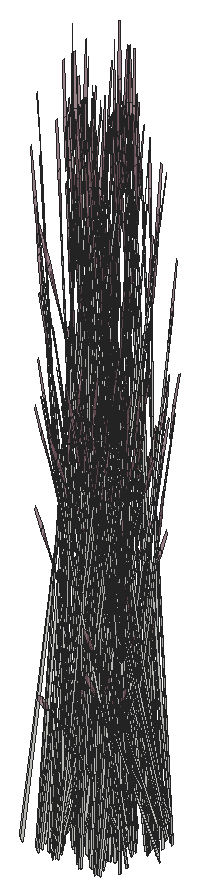
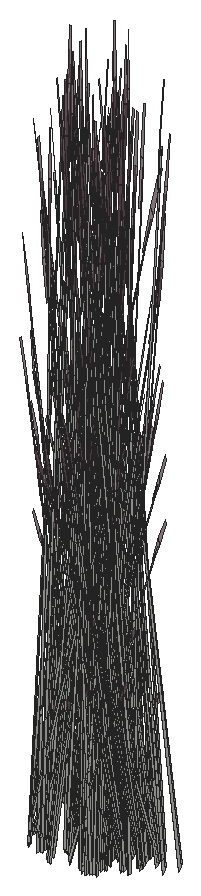
# SketchUp Ruby script. Lengths in inches.
U = 1.inch
M = Sketchup.active_model
def pt(a) = Geom::Point3d.new(a.map { |v| v * U })
def face(e, loops, mat)
  f = e.add_face(loops[0].map { |a| pt(a) })
  loops[1..].each { |l| e.add_face(l.map { |a| pt(a) }).erase! }
  f.material = f.back_material = mat if mat
  f
end
# faces: each face lists its corners as indices into pts; further lists are holes
def faces(e, pts, list, mat = nil) = list.each { |f| face(e, (f[0].is_a?(Array) ? f : [f]).map { |l| l.map { |i| pts[i] } }, mat) }
# xy, xz, yz: faces in a plane at the given z, y or x. An outline is a flat list of corners, or four numbers for a rectangle; further outlines are holes
def ring(l) = l.size == 4 ? [[l[0], l[1]], [l[2], l[1]], [l[2], l[3]], [l[0], l[3]]] : l.each_slice(2).to_a
def flat(e, list, mat, &to3) = list.each { |f| face(e, (f[0].is_a?(Array) ? f : [f]).map { |l| ring(l).map { |u, v| to3.(u, v) } }, mat) }
def xy(e, z, list, mat = nil) = flat(e, list, mat) { |x, y| [x, y, z] }
def xz(e, y, list, mat = nil) = flat(e, list, mat) { |x, z| [x, y, z] }
def yz(e, x, list, mat = nil) = flat(e, list, mat) { |y, z| [x, y, z] }
def lines(e, pts, list) = list.each { |a, b| e.add_line(pt(pts[a]), pt(pts[b])) }
# prism: a flat outline (further loops are holes) pulled along v
def prism(e, loops, v, mat = nil)
  f = face(e, loops, mat); d = Geom::Vector3d.new(v.map { |x| x * U })
  f.pushpull(f.normal.samedirection?(d) ? d.length : -d.length)
end
def box(e, o, s, mat = nil) = prism(e, [[o, [o[0] + s[0], o[1], o[2]], [o[0] + s[0], o[1] + s[1], o[2]], [o[0], o[1] + s[1], o[2]]]], [0, 0, s[2]], mat)
def at(x, y, z, deg = 0) = Geom::Transformation.translation(pt([x, y, z])) * Geom::Transformation.rotation(ORIGIN, Z_AXIS, deg.degrees)
def axes(o, x, y, z) = Geom::Transformation.new([*x, 0, *y, 0, *z, 0, *pt(o).to_a, 1])
def part(name) = M.definitions.add(name)
# library, detail: a bought-in or finely detailed component or shape, given as its bounding box
def library(name, o, s) = part(name).tap { |d| box(d.entities, o, s) }
def detail(e, o, s) = box(e.add_group.entities, o, s)
def put(e, d, t, mat = nil) = e.add_instance(d, t).tap { |i| i.material = mat if mat }
def group(e, t, mat = nil) = e.add_group.tap { |g| g.transformation = t; g.material = mat if mat }.entities
root = M.entities
M.materials.add("LightPink_Translucent").color = [144, 107, 117]
M.materials["LightPink_Translucent"].alpha = 0.75
c1 = part("blade")
p = [[2.15,0.21,22],[0,0.17,0],[0.09,0.45,0],[2.18,0.31,22],[2.29,0.31,22],[0.38,0.45,0],
  [2.48,0.24,33],[2.49,0.24,33],[2.48,0.22,33]]
faces(c1.entities,p,[[0,1,2,3],[4,5,2,3],[6,3,4,7],[8,0,3,6]])
c2 = part("seeds")
p = [[0.3,-0.1,1.38],[-0.01,-0.03,1.59],[-0.01,-0.03,0.03],[0.14,-0.07,-0.07],[0.29,-0.03,3],[0.15,0.01,3.11]]
faces(c2.entities,p,[[0,1,2,3],[1,0,4,5]],"LightPink_Translucent")
c3 = part("blade with seeds")
put(c3.entities,c1,at(0,0,0))
put(c3.entities,c2,axes([2.4,0.25,30.99],[1.5799,-0.05474,1.17369],[-0.12525,1.92788,0.29478],[-0.07173,-0.02425,1.56792]))
put(root,c3,axes([356.83,652.4,625.22],[-0.1064,0.35863,0.35414],[-0.31043,-0.1046,-0.4572],[-0.02846,-0.14439,0.87481]))
put(root,c3,axes([350.33,651.97,625.26],[-0.17758,-0.42229,-0.1216],[0.31518,-0.20752,-0.67495],[0.13282,-0.05572,1.02557]))
put(root,c3,axes([350.32,651.6,624.91],[0.09562,-0.42421,-0.51099],[0.32782,0.1454,-0.3958],[0.13199,-0.0389,0.97773]))
put(root,c3,axes([352.76,650.92,621.17],[0.32928,0.11539,-0.30978],[-0.08291,0.40636,0.30978],[0.06638,-0.04686,1.38974]))
put(root,c3,axes([349.8,649.875,622.6],[0.22066,-0.46731,0],[0.36918,0.26061,-0.51607],[0.08408,0.05936,1.63711]))
put(root,c3,axes([355.87,652.46,624.85],[-0.34827,0.11086,-0.51099],[-0.06092,-0.41983,-0.3958],[-0.09354,-0.12031,0.97773]))
put(root,c3,axes([356.11,652.09,625.6],[-0.23555,0.44708,-0.13619],[-0.34112,-0.25757,-0.75594],[-0.11858,-0.12631,1.14864]))
put(root,c3,axes([350.67,651.72,622.21],[-0.22732,0.05597,1.41583],[-0.03618,-0.44548,0.08104],[0.15921,-0.06743,0.80566]))
put(root,c3,axes([351.08,651.33,622.49],[-0.21881,-0.29821,-0.06488],[0.23965,-0.27324,-0.29416],[0.0679,-0.01924,0.97024]))
put(root,c3,axes([351.52,652.2,624.73],[-0.17758,-0.42229,-0.1216],[0.31518,-0.20752,-0.67495],[0.13282,-0.05572,1.02557]))
put(root,c3,axes([351.51,651.84,624.37],[0.09562,-0.42421,-0.51099],[0.32782,0.1454,-0.3958],[0.13199,-0.0389,0.97773]))
put(root,c3,axes([350.99,650.11,622.07],[0.22066,-0.46731,0],[0.36918,0.26061,-0.51607],[0.08408,0.05936,1.63711]))
put(root,c3,axes([354.65,651.92,623.87],[0.2423,0.19613,0.0643],[-0.14107,0.2793,0.50621],[0.07768,-0.0903,0.77189]))
put(root,c3,axes([354.58,651.84,623.87],[0.08753,0.42921,0.48003],[-0.34336,0.07449,0.3958],[0.1012,-0.10094,0.9933]))
put(root,c3,axes([356.42,651.83,622.3],[-0.2439,0.26754,-0.03893],[-0.22348,-0.29302,-0.17649],[-0.01573,-0.08303,0.58215]))
put(root,c3,axes([350.25,651.76,625.21],[0.31014,-0.20596,-0.71045],[0.17284,0.42397,0.08574],[0.14985,-0.04816,1.00501]))
put(root,c3,axes([351.86,651.96,621.67],[-0.22732,0.05597,1.41583],[-0.03618,-0.44548,0.08104],[0.15921,-0.06743,0.80566]))
put(root,c3,axes([352.27,651.57,621.95],[-0.21881,-0.29821,-0.06488],[0.23965,-0.27324,-0.29416],[0.0679,-0.01924,0.97024]))
put(root,c3,axes([358.3,652.55,625.55],[-0.00658,0.0559,1.77383],[-0.32474,0.20287,-0.16761],[-0.09556,-0.1037,0.31391]))
put(root,c3,axes([351.83,652.33,621.47],[-0.32829,0.39208,0.30756],[-0.32849,-0.38796,-0.36492],[-0.01146,-0.11134,1.64885]))
put(root,c3,axes([355.21,651.96,624.88],[-0.07594,-0.00329,1.74944],[-0.24177,0.32918,-0.27667],[-0.129,-0.06726,0.14031]))
put(root,c3,axes([350.8,650.36,622.17],[-0.33032,-0.23318,0.49651],[0.19744,-0.41812,0],[0.07523,0.05311,1.57504]))
put(root,c3,axes([351.45,652,624.67],[0.31014,-0.20596,-0.71045],[0.17284,0.42397,0.08574],[0.14985,-0.04816,1.00501]))
put(root,c3,axes([350.21,651.84,625.28],[-0.29332,-0.1301,0.35414],[0.08555,-0.37955,-0.4572],[0.11809,-0.0348,0.87481]))
put(root,c3,axes([352.87,652.52,621.57],[0.39767,0.22603,0.24065],[-0.19139,0.46966,0.50002],[0,-0.10827,1.60543]))
put(root,c3,axes([352.72,653.15,621.58],[0.09355,-0.55261,-0.23429],[0.44354,0.09633,0.51271],[-0.0775,-0.07631,1.5644]))
put(root,c3,axes([356.73,655,623.49],[0.305,0.18805,1.51261],[-0.29879,0.40513,0.59816],[-0.13384,-0.24012,1.26806]))
put(root,c3,axes([348.2,650.71,621.82],[-0.3474,0.18671,1.28929],[-0.11057,-0.53572,0.50096],[0.21332,0.00891,1.46642]))
put(root,c3,axes([356.09,652.46,625.22],[0.05451,0.37564,0.35414],[-0.31161,0.09919,-0.4572],[-0.0837,-0.10765,0.87481]))
put(root,c3,axes([355.13,653.7,622.1875],[0,-0.46636,-0.49651],[0.39487,0,0],[0,-0.10622,1.57504]))
put(root,c3,axes([355.15,652.7,625.26],[0.29147,-0.34417,0.53763],[0.25138,0.3655,0.4433],[-0.13675,-0.06349,1.11249]))
put(root,c3,axes([358.29,653.98,625.83],[-0.30095,-0.22541,-0.71045],[0.21388,-0.395,0.08574],[-0.10904,-0.13459,1.00501]))
put(root,c3,axes([350.91,651.43,621.72],[-0.01845,-0.0708,1.76342],[0.12793,-0.41416,-0.26939],[0.12905,-0.00596,0.30037]))
put(root,c3,axes([358.1875,653.68,625.37],[-0.05451,-0.37564,-0.35414],[0.31161,-0.09919,0.4572],[-0.0837,-0.10765,0.87481]))
put(root,c3,axes([351.4,652.08,624.74],[-0.29332,-0.1301,0.35414],[0.08555,-0.37955,-0.4572],[0.11809,-0.0348,0.87481]))
put(root,c3,axes([349.39,650.94,621.28],[-0.3474,0.18671,1.28929],[-0.11057,-0.53572,0.50096],[0.21332,0.00891,1.46642]))
put(root,c3,axes([352.74,652.2,621.86],[-0.38326,0.02879,0.44739],[-0.03466,-0.47788,-0.21531],[0.06861,-0.04843,1.43643]))
put(root,c3,axes([350.33,651.08,622.31],[0.06809,-0.4162,0.1448],[0.33266,0.07225,-0.41347],[0.06054,0.04274,1.26744]))
put(root,c3,axes([351.75,652.55,621.62],[0,0.46636,0.49651],[-0.39487,0,0],[0,-0.10622,1.57504]))
put(root,c3,axes([354.54,653.02,624.17],[-0.17758,-0.42229,-0.1216],[0.31518,-0.20752,-0.67495],[0.13282,-0.05572,1.02557]))
put(root,c3,axes([352.11,651.67,621.18],[-0.01845,-0.0708,1.76342],[0.12793,-0.41416,-0.26939],[0.12905,-0.00596,0.30037]))
put(root,c3,axes([354.01,650.93,621.51],[0.22066,-0.46731,0],[0.36918,0.26061,-0.51607],[0.08408,0.05936,1.63711]))
put(root,c3,axes([352.6875,652.93,621.35],[-0.21202,-0.39143,-0.44739],[0.32115,-0.27564,0.21531],[-0.06861,-0.04843,1.43643]))
put(root,c3,axes([352.73,652.375,621.5],[0.15345,0.52148,0.45755],[-0.43845,0.18134,0.17955],[0.00536,-0.09582,1.58856]))
put(root,c3,axes([349.1,650.98,622.89],[0.35635,-0.30962,-0.29095],[0.23697,0.43749,-0.50002],[0.08792,0.04443,1.59708]))
put(root,c3,axes([350.52,651.8,624.75],[0.29332,0.1301,-0.35414],[-0.08555,0.37955,0.4572],[0.11809,-0.0348,0.87481]))
put(root,c3,axes([350.19,651.19,622.41],[-0.21202,-0.39143,0.44739],[0.32115,-0.27564,-0.21531],[0.06861,0.04843,1.43643]))
put(root,c3,axes([355.28,652.7,624.9],[0.01777,-0.35463,0.0643],[0.26836,0.00972,0.50621],[-0.1028,-0.03711,0.77189]))
put(root,c3,axes([357.7,653.61,622.34],[-0.03419,0.06144,1.76342],[-0.3455,0.13246,-0.26939],[-0.08346,-0.12049,0.30037]))
put(root,c3,axes([350,650.16,622.24],[0.33032,0.23318,-0.49651],[-0.19744,0.41812,0],[0.07523,0.05311,1.57504]))
put(root,c3,axes([355.29,652.38,621.4],[-0.21881,-0.29821,-0.06488],[0.23965,-0.27324,-0.29416],[0.0679,-0.01924,0.97024]))
put(root,c3,axes([356.21,653.89,622.38],[0.17124,-0.42022,-0.44739],[0.35581,0.20224,0.21531],[0,-0.09687,1.43643]))
put(root,c3,axes([355.18,652.8125,624.7],[-0.20082,-0.29199,-0.35414],[0.2293,-0.2764,0.4572],[-0.1165,-0.04206,0.87481]))
put(root,c3,axes([352.65,652.78,621.86],[-0.17124,0.42022,0.44739],[-0.35581,-0.20224,-0.21531],[0,-0.09687,1.43643]))
put(root,c3,axes([353.28,652.42,621.34],[0,-0.53961,0],[0.44133,0,0],[0,0,1.79456]))
put(root,c3,axes([355.3,653.71,622.2],[0.24637,-0.29097,-0.30978],[0.24637,0.29097,0.30978],[0,-0.09372,1.38974]))
put(root,c3,axes([357.52,654.22,624.72],[0.1311,0.08035,1.71376],[-0.27131,0.33708,0.13857],[-0.16909,-0.15206,0.73262]))
put(root,c3,axes([350.29,651.22,622.36],[0.35635,-0.30962,-0.29095],[0.23697,0.43749,-0.50002],[0.08792,0.04443,1.59708]))
put(root,c3,axes([351.71,652.03,624.22],[0.29332,0.1301,-0.35414],[-0.08555,0.37955,0.4572],[0.11809,-0.0348,0.87481]))
put(root,c3,axes([353.82,651.17,621.62],[-0.33032,-0.23318,0.49651],[0.19744,-0.41812,0],[0.07523,0.05311,1.57504]))
put(root,c3,axes([355.2,652.32,622.3],[-0.10181,0.3808,-0.03893],[-0.31336,-0.11714,-0.17649],[-0.04758,-0.06228,0.58215]))
put(root,c3,axes([356.17,654.24,622.83],[-0.39748,-0.22252,-0.29095],[0.19139,-0.46966,-0.50002],[-0.01249,-0.11531,1.59708]))
put(root,c3,axes([349.72,651.33,624.1],[-0.14639,0.01056,1.71376],[0.09712,-0.45778,0.13857],[0.20862,0.02831,0.73262]))
put(root,c3,axes([351.19,650.4,621.71],[0.33032,0.23318,-0.49651],[-0.19744,0.41812,0],[0.07523,0.05311,1.57504]))
put(root,c3,axes([349.91,650.33,622.25],[0.08291,0.40636,-0.30978],[-0.32928,0.11539,0.30978],[0.06638,0.04686,1.38974]))
put(root,c3,axes([355.03,654.05,622.54],[-0.44133,0,0],[0,-0.52122,-0.51607],[0,-0.11871,1.63711]))
put(root,c3,axes([350.57,651.73,621.9],[0.39487,0,0],[0,0.48281,0],[0,0,1.78407]))
put(root,c3,axes([353.07,652.08,621.5],[-0.29264,0.42323,0.45755],[-0.34767,-0.3736,0.17955],[0.07055,-0.04224,1.58856]))
put(root,c3,axes([355.11,653.125,622.76],[0.06891,0.12984,1.43002],[-0.15879,0.35293,-0.30754],[-0.16304,-0.08436,0.61141]))
put(root,c3,axes([358.15,653.99,625.53],[-0.34827,0.11086,-0.51099],[-0.06092,-0.41983,-0.3958],[-0.09354,-0.12031,0.97773]))
put(root,c3,axes([350.47,651.96,624.96],[0.12963,0.31798,0.0643],[-0.23638,0.15564,0.50621],[0.1042,-0.03071,0.77189]))
put(root,c3,axes([358.39,653.61,626.28],[-0.23555,0.44708,-0.13619],[-0.34112,-0.25757,-0.75594],[-0.11858,-0.12631,1.14864]))
put(root,c3,axes([353.39,652.84,621.44],[-0.32829,-0.4014,-0.06131],[0.32849,-0.40164,0],[-0.01146,-0.01402,1.75571]))
put(root,c3,axes([350.45,651.84,624.96],[-0.09971,0.42522,0.48003],[-0.32782,-0.1454,0.3958],[0.12892,-0.02555,0.9933]))
put(root,c3,axes([352.56,651.38,621.61],[-0.10196,0.46348,0.17642],[-0.3731,-0.13116,0.35086],[0.06445,-0.00226,1.60407]))
put(root,c3,axes([355.39,653.01,625.15],[-0.35281,-0.01123,-0.71045],[0.0237,-0.47284,0.08574],[-0.14947,-0.0499,1.00501]))
put(root,c3,axes([354.42,652.89,624.1875],[-0.29332,-0.1301,0.35414],[0.08555,-0.37955,-0.4572],[0.11809,-0.0348,0.87481]))
put(root,c3,axes([350.91,651.57,623.57],[-0.14639,0.01056,1.71376],[0.09712,-0.45778,0.13857],[0.20862,0.02831,0.73262]))
put(root,c3,axes([351.1,650.57,621.72],[0.08291,0.40636,-0.30978],[-0.32928,0.11539,0.30978],[0.06638,0.04686,1.38974]))
put(root,c3,axes([352.41,651.76,620.73],[-0.3474,0.18671,1.28929],[-0.11057,-0.53572,0.50096],[0.21332,0.00891,1.46642]))
put(root,c3,axes([353.34,651.9,621.75],[0.06809,-0.4162,0.1448],[0.33266,0.07225,-0.41347],[0.06054,0.04274,1.26744]))
put(root,c3,axes([351.67,652.19,624.42],[0.12963,0.31798,0.0643],[-0.23638,0.15564,0.50621],[0.1042,-0.03071,0.77189]))
put(root,c3,axes([352.77,652.89,621.5],[0.44609,0.09826,0.45755],[-0.09078,0.55493,0.17955],[-0.06519,-0.05359,1.58856]))
put(root,c3,axes([351.64,652.08,624.42],[-0.09971,0.42522,0.48003],[-0.32782,-0.1454,0.3958],[0.12892,-0.02555,0.9933]))
put(root,c3,axes([353.2,652.01,621.86],[-0.21202,-0.39143,0.44739],[0.32115,-0.27564,-0.21531],[0.06861,0.04843,1.43643]))
put(root,c3,axes([349.52,651.05,622.28],[0.36714,0.07646,-0.62353],[-0.07747,0.47163,-0.16365],[0.10956,0.05715,1.37633]))
put(root,c3,axes([351.14,651.875,622.99],[-0.21807,0.07699,1.1486],[0.10265,-0.31819,0.84392],[0.11568,0.02177,0.25299]))
put(root,c3,axes([357.49,653.48,625.56],[-0.07594,-0.00329,1.74944],[-0.24177,0.32918,-0.27667],[-0.129,-0.06726,0.14031]))
put(root,c3,axes([350.51,652.79,621.875],[0.37054,-0.15823,-0.19198],[0.1302,0.45581,0.00008],[0.0409,-0.01749,1.73897]))
put(root,c3,axes([355.375,653.92,622.5],[-0.32829,0.39208,0.30756],[-0.32849,-0.38796,-0.36492],[-0.01146,-0.11134,1.64885]))
put(root,c3,axes([354.92,652.24,624.88],[0.02617,0.04654,1.77383],[-0.12614,0.41836,-0.16761],[-0.12775,0.00303,0.31391]))
put(root,c3,axes([352.53,653.77,621.61],[0.37926,-0.12378,0.17642],[0.09365,0.46065,0.35086],[-0.03382,-0.06712,1.60407]))
put(root,c3,axes([353.31,652.03,621.8],[0.35635,-0.30962,-0.29095],[0.23697,0.43749,-0.50002],[0.08792,0.04443,1.59708]))
put(root,c3,axes([350.71,651.29,621.75],[0.36714,0.07646,-0.62353],[-0.07747,0.47163,-0.16365],[0.10956,0.05715,1.37633]))
put(root,c3,axes([352.33,652.11,622.46],[-0.21807,0.07699,1.1486],[0.10265,-0.31819,0.84392],[0.11568,0.02177,0.25299]))
put(root,c3,axes([351.04,653.22,624.93],[-0.03191,-0.04083,1.77383],[0.06981,-0.43764,-0.16761],[0.12571,-0.02796,0.31391]))
put(root,c3,axes([356.27,654.73,622.61],[0.09355,-0.55261,-0.23429],[0.44354,0.09633,0.51271],[-0.0775,-0.07631,1.5644]))
put(root,c3,axes([354.21,651.21,621.16],[0.33032,0.23318,-0.49651],[-0.19744,0.41812,0],[0.07523,0.05311,1.57504]))
put(root,c3,axes([355.28,653.1,624.85],[-0.25628,0.30892,-0.51099],[-0.22444,-0.32634,-0.3958],[-0.13021,-0.047,0.97773]))
put(root,c3,axes([353.58,652.54,621.34],[0.39487,0,0],[0,0.48281,0],[0,0,1.78407]))
put(root,c3,axes([357.4375,654.23,625.9375],[0.29147,-0.34417,0.53763],[0.25138,0.3655,0.4433],[-0.13675,-0.06349,1.11249]))
put(root,c3,axes([355.47,652.97,625.22],[0.20082,0.29199,0.35414],[-0.2293,0.2764,-0.4572],[-0.1165,-0.04206,0.87481]))
put(root,c3,axes([353.69,651.41,621.61],[-0.37926,0.12378,0.17642],[-0.09365,-0.46065,0.35086],[0.03382,0.06712,1.60407]))
put(root,c3,axes([350.76,652.86,624.15],[-0.06755,-0.39203,-0.03492],[0.31928,-0.09013,-0.15832],[0.06667,0.02485,0.52218]))
put(root,c3,axes([354.7,653.51,622.93],[0.22533,-0.03337,1.1486],[-0.14293,0.29403,0.84392],[-0.11135,-0.04411,0.25299]))
put(root,c3,axes([349.93,652.84,625.26],[0.0189,-0.47427,-0.1216],[0.35781,0.01296,-0.67495],[0.13781,0.03295,1.02557]))
put(root,c3,axes([352.23,653.46,624.4],[-0.03191,-0.04083,1.77383],[0.06981,-0.43764,-0.16761],[0.12571,-0.02796,0.31391]))
put(root,c3,axes([354.12,651.38,621.17],[0.08291,0.40636,-0.30978],[-0.32928,0.11539,0.30978],[0.06638,0.04686,1.38974]))
put(root,c3,axes([355.41,652.78,625.2],[-0.0189,0.47427,-0.1216],[-0.35781,-0.01296,-0.67495],[-0.13781,-0.03295,1.02557]))
put(root,c3,axes([355.3,654.13,622.65],[0,0.46636,0.49651],[-0.39487,0,0],[0,-0.10622,1.57504]))
put(root,c3,axes([350.52,651.4375,621.9],[0.21202,0.39143,-0.44739],[-0.32115,0.27564,0.21531],[0.06861,0.04843,1.43643]))
put(root,c3,axes([349.88,652.66,625.28],[-0.20082,-0.29199,0.35414],[0.2293,-0.2764,-0.4572],[0.1165,0.04206,0.87481]))
put(root,c3,axes([354.68,653.01,623.87],[0.12963,0.31798,0.0643],[-0.23638,0.15564,0.50621],[0.1042,-0.03071,0.77189]))
put(root,c3,axes([351.95,653.09,623.62],[-0.06755,-0.39203,-0.03492],[0.31928,-0.09013,-0.15832],[0.06667,0.02485,0.52218]))
put(root,c3,axes([351.125,653.08,624.73],[0.0189,-0.47427,-0.1216],[0.35781,0.01296,-0.67495],[0.13781,0.03295,1.02557]))
put(root,c3,axes([354.96,653.43,624.04],[0.14639,-0.01056,1.71376],[-0.09712,0.45778,0.13857],[-0.20862,-0.02831,0.73262]))
put(root,c3,axes([353.45,652.29,621.52],[-0.44609,-0.09826,0.49198],[0.09078,-0.55493,0.19306],[0.06519,0.05359,1.70813]))
put(root,c3,axes([356.23,654.51,622.38],[-0.21202,-0.39143,-0.44739],[0.32115,-0.27564,0.21531],[-0.06861,-0.04843,1.43643]))
put(root,c3,axes([356.28,653.96,622.53],[0.15345,0.52148,0.45755],[-0.43845,0.18134,0.17955],[0.00536,-0.09582,1.58856]))
put(root,c3,axes([354.66,652.89,623.87],[-0.09971,0.42522,0.48003],[-0.32782,-0.1454,0.3958],[0.12892,-0.02555,0.9933]))
put(root,c3,axes([357.57,654.23,625.58],[0.01777,-0.35463,0.0643],[0.26836,0.00972,0.50621],[-0.1028,-0.03711,0.77189]))
put(root,c3,axes([353.1,653.66,621.34],[-0.11516,-0.40207,0],[0.32884,-0.1408,0],[0,0,1.54371]))
put(root,c3,axes([351.45,651.81,622.17],[0,-0.46636,0.49651],[0.39487,0,0],[0,0.10622,1.57504]))
put(root,c3,axes([350.73,652.39,622.82],[-0.085,-0.1147,1.43002],[0.1106,-0.37943,-0.30754],[0.17198,0.0514,0.61141]))
put(root,c3,axes([352.88,653.28,621.75],[-0.06809,0.4162,0.1448],[-0.33266,-0.07225,-0.41347],[-0.06054,-0.04274,1.26744]))
put(root,c3,axes([357.47,654.34,625.37],[-0.20082,-0.29199,-0.35414],[0.2293,-0.2764,0.4572],[-0.1165,-0.04206,0.87481]))
put(root,c3,axes([350.7,651.68,622.31],[0.32884,-0.136,0.1448],[0.11516,0.38837,-0.41347],[0,0.08547,1.26744]))
put(root,c3,axes([353.53,653.61,621.32],[0.37054,-0.15823,-0.19198],[0.1302,0.45581,0.00008],[0.0409,-0.01749,1.73897]))
put(root,c3,axes([356.2,654.37,622.89],[-0.17124,0.42022,0.44739],[-0.35581,-0.20224,-0.21531],[0,-0.09687,1.43643]))
put(root,c3,axes([351.07,652.9,624.74],[-0.20082,-0.29199,0.35414],[0.2293,-0.2764,-0.4572],[0.1165,0.04206,0.87481]))
put(root,c3,axes([353.66,653.8,621.61],[0.10196,-0.46348,0.17642],[0.3731,0.13116,0.35086],[-0.06445,0.00226,1.60407]))
put(root,c3,axes([357.49,653.84,622.97],[-0.10181,0.3808,-0.03893],[-0.31336,-0.11714,-0.17649],[-0.04758,-0.06228,0.58215]))
put(root,c3,axes([353.57,652.75,621.35],[0.24637,0.30123,0],[-0.24637,0.30123,0],[0,0,1.69266]))
put(root,c3,axes([351.92,652.62,622.28],[-0.085,-0.1147,1.43002],[0.1106,-0.37943,-0.30754],[0.17198,0.0514,0.61141]))
put(root,c3,axes([354.24,652.61,621.61],[-0.2773,-0.3397,0.17642],[0.27945,-0.32949,0.35086],[-0.03063,0.06937,1.60407]))
put(root,c3,axes([357.32,655.58,623.22],[-0.44133,0,0],[0,-0.52122,-0.51607],[0,-0.11871,1.63711]))
put(root,c3,axes([350.24,652.56,624.94],[0.07571,-0.00789,1.74944],[0.20767,-0.36231,-0.27667],[0.13467,0.04783,0.14031]))
put(root,c3,axes([353.73,652.1,621.2],[0.36714,0.07646,-0.62353],[-0.07747,0.47163,-0.16365],[0.10956,0.05715,1.37633]))
put(root,c3,axes([357.39,654.65,623.4375],[0.06891,0.12984,1.43002],[-0.15879,0.35293,-0.30754],[-0.16304,-0.08436,0.61141]))
put(root,c3,axes([356.04,654.66,622.23],[-0.36714,-0.07646,-0.62353],[0.07747,-0.47163,-0.16365],[-0.10956,-0.05715,1.37633]))
put(root,c3,axes([353.02,653.84,621.33],[-0.35581,-0.20937,0],[0.17124,-0.43505,0],[0,0,1.62707]))
put(root,c3,axes([353.3125,653.29,621.6],[-0.34464,-0.37536,-0.25192],[0.29,-0.42149,0.5513],[-0.0928,0.04391,1.68216]))
put(root,c3,axes([352.41,654.01,621.62],[0.33032,0.23318,0.49651],[-0.19744,0.41812,0],[-0.07523,-0.05311,1.57504]))
put(root,c3,axes([356.94,654.42,622.47],[-0.32829,-0.4014,-0.06131],[0.32849,-0.40164,0],[-0.01146,-0.01402,1.75571]))
put(root,c3,axes([357.68,654.53,625.83],[-0.35281,-0.01123,-0.71045],[0.0237,-0.47284,0.08574],[-0.14947,-0.0499,1.00501]))
put(root,c3,axes([351.4375,652.8,624.41],[0.07571,-0.00789,1.74944],[0.20767,-0.36231,-0.27667],[0.13467,0.04783,0.14031]))
put(root,c3,axes([353.57,652.39,621.86],[0.17124,-0.42022,0.44739],[0.35581,0.20224,-0.21531],[0,0.09687,1.43643]))
put(root,c3,axes([349.95,652.62,625.21],[0.35281,0.01123,-0.71045],[-0.0237,0.47284,0.08574],[0.14947,0.0499,1.00501]))
put(root,c3,axes([354.9,653.78,624.9],[0.09971,-0.42522,0.48003],[0.32782,0.1454,0.3958],[-0.12892,0.02555,0.9933]))
put(root,c3,axes([353.5,652.63,621.43],[0,0.53934,-0.05637],[-0.44133,0,0],[0,0.01695,1.79368]))
put(root,c3,axes([354.87,653.67,624.9],[-0.12963,-0.31798,0.0643],[0.23638,-0.15564,0.50621],[-0.1042,0.03071,0.77189]))
put(root,c3,axes([353.54,652.25,621.35],[0.21202,0.39143,-0.44739],[-0.32115,0.27564,0.21531],[0.06861,0.04843,1.43643]))
put(root,c3,axes([356.32,654.47,622.53],[0.44609,0.09826,0.45755],[-0.09078,0.55493,0.17955],[-0.06519,-0.05359,1.58856]))
put(root,c3,axes([354.97,653.91,623.07],[-0.06755,-0.39203,-0.03492],[0.31928,-0.09013,-0.15832],[0.06667,0.02485,0.52218]))
put(root,c3,axes([354.14,653.89,624.17],[0.0189,-0.47427,-0.1216],[0.35781,0.01296,-0.67495],[0.13781,0.03295,1.02557]))
put(root,c3,axes([354.86,653.99,621.66],[0.00895,0.0735,1.76342],[-0.18044,0.38382,-0.26939],[-0.12817,-0.01935,0.30037]))
put(root,c3,axes([351.14,652.85,624.67],[0.35281,0.01123,-0.71045],[-0.0237,0.47284,0.08574],[0.14947,0.0499,1.00501]))
put(root,c3,axes([354.47,652.63,621.62],[0,-0.46636,0.49651],[0.39487,0,0],[0,0.10622,1.57504]))
put(root,c3,axes([353.48,652.98,621.86],[0.38326,-0.02879,0.44739],[0.03466,0.47788,-0.21531],[-0.06861,0.04843,1.43643]))
put(root,c3,axes([350.53,651.66,622.6],[0.44133,0,0],[0,0.52122,-0.51607],[0,0.11871,1.63711]))
put(root,c3,axes([355.65,655.38,622.2],[-0.08291,-0.40636,-0.30978],[0.32928,-0.11539,0.30978],[-0.06638,-0.04686,1.38974]))
put(root,c3,axes([353.72,652.49,621.75],[0.32884,-0.136,0.1448],[0.11516,0.38837,-0.41347],[0,0.08547,1.26744]))
put(root,c3,axes([357.2,653.76,625.55],[0.02617,0.04654,1.77383],[-0.12614,0.41836,-0.16761],[-0.12775,0.00303,0.31391]))
put(root,c3,axes([354.09,653.71,624.1875],[-0.20082,-0.29199,0.35414],[0.2293,-0.2764,-0.4572],[0.1165,0.04206,0.87481]))
put(root,c3,axes([353.14,653.21,621.35],[-0.38326,0.02879,-0.44739],[-0.03466,-0.47788,0.21531],[-0.06861,0.04843,1.43643]))
put(root,c3,axes([350.16,652.8125,624.75],[0.20082,0.29199,-0.35414],[-0.2293,0.2764,0.4572],[0.1165,0.04206,0.87481]))
put(root,c3,axes([356.08,655.35,622.64],[0.37926,-0.12378,0.17642],[0.09365,0.46065,0.35086],[-0.03382,-0.06712,1.60407]))
put(root,c3,axes([350.06,652.92,624.96],[-0.01777,0.35463,0.0643],[-0.26836,-0.00972,0.50621],[0.1028,0.03711,0.77189]))
put(root,c3,axes([351.72,651.89,622.07],[0.44133,0,0],[0,0.52122,-0.51607],[0,0.11871,1.63711]))
put(root,c3,axes([357.5625,654.63,625.53],[-0.25628,0.30892,-0.51099],[-0.22444,-0.32634,-0.3958],[-0.13021,-0.047,0.97773]))
put(root,c3,axes([355.5625,655.55,622.1875],[-0.33032,-0.23318,-0.49651],[0.19744,-0.41812,0],[-0.07523,-0.05311,1.57504]))
put(root,c3,axes([354.83,653.83,624.7],[-0.29332,-0.1301,-0.35414],[0.08555,-0.37955,0.4572],[-0.11809,0.0348,0.87481]))
put(root,c3,axes([357.75,654.49,625.9],[0.20082,0.29199,0.35414],[-0.2293,0.2764,-0.4572],[-0.1165,-0.04206,0.87481]))
put(root,c3,axes([350.08,652.81,624.96],[-0.26024,0.30729,0.48003],[-0.22444,-0.32634,0.3958],[0.1221,0.05668,0.9933]))
put(root,c3,axes([350.59,651.71,622.36],[0.39748,0.22252,-0.29095],[-0.19139,0.46966,-0.50002],[0.01249,0.11531,1.59708]))
put(root,c3,axes([353.42,653.85,621.34],[0.35581,0.20937,0],[-0.17124,0.43505,0],[0,0,1.74954]))
put(root,c3,axes([356.98,655.04,623.61],[0.22533,-0.03337,1.1486],[-0.14293,0.29403,0.84392],[-0.11135,-0.04411,0.25299]))
put(root,c3,axes([356.46,654.73,622.83],[-0.35635,0.30962,-0.29095],[-0.23697,-0.43749,-0.50002],[-0.08792,-0.04443,1.59708]))
put(root,c3,axes([351.36,653.05,624.22],[0.20082,0.29199,-0.35414],[-0.2293,0.2764,0.4572],[0.1165,0.04206,0.87481]))
put(root,c3,axes([351.45,652.24,621.72],[-0.24637,0.29097,-0.30978],[-0.24637,-0.29097,0.30978],[0,0.09372,1.38974]))
put(root,c3,axes([351.25,653.16,624.42],[-0.01777,0.35463,0.0643],[-0.26836,-0.00972,0.50621],[0.1028,0.03711,0.77189]))
put(root,c3,axes([357.7,654.31,625.88],[-0.0189,0.47427,-0.1216],[-0.35781,-0.01296,-0.67495],[-0.13781,-0.03295,1.02557]))
put(root,c3,axes([353.5625,654.32,621.33],[-0.21791,-0.46895,-0.05142],[0.36918,-0.26061,0.51607],[-0.09097,0.04465,1.6363]))
put(root,c3,axes([353.49,653.18,621.75],[0.26075,0.2802,0.1448],[-0.2175,0.31612,-0.41347],[-0.06054,0.04274,1.26744]))
put(root,c3,axes([351.28,653.05,624.42],[-0.26024,0.30729,0.48003],[-0.22444,-0.32634,0.3958],[0.1221,0.05668,0.9933]))
put(root,c3,axes([357.24,654.96,624.72],[0.14639,-0.01056,1.71376],[-0.09712,0.45778,0.13857],[-0.20862,-0.02831,0.73262]))
put(root,c3,axes([349.44,652.0625,624.1],[-0.1311,-0.08035,1.71376],[0.27131,-0.33708,0.13857],[0.16909,0.15206,0.73262]))
put(root,c3,axes([356.65,655.25,622.37],[-0.11516,-0.40207,0],[0.32884,-0.1408,0],[0,0,1.54371]))
put(root,c3,axes([356.43,654.86,622.79],[-0.06809,0.4162,0.1448],[-0.33266,-0.07225,-0.41347],[-0.06054,-0.04274,1.26744]))
put(root,c3,axes([355.14,653.78,625.22],[0.29332,0.1301,0.35414],[-0.08555,0.37955,-0.4572],[-0.11809,0.0348,0.87481]))
put(root,c3,axes([353.76,654.05,621.62],[0.33032,-0.23318,0.49651],[0.19744,0.41812,0],[-0.07523,0.05311,1.57504]))
put(root,c3,axes([357.21,655.38,622.64],[0.10196,-0.46348,0.17642],[0.3731,0.13116,0.35086],[-0.06445,0.00226,1.60407]))
put(root,c3,axes([350.45,653.4,624.74],[-0.05451,-0.37564,0.35414],[0.31161,-0.09919,-0.4572],[0.0837,0.10765,0.87481]))
put(root,c3,axes([353.29,653.68,621.43],[0.15345,0.53576,-0.06012],[-0.43845,0.18773,0],[0.00536,0.01871,1.72173]))
put(root,c3,axes([351.62,652.25,621.71],[0,0.46636,-0.49651],[-0.39487,0,0],[0,0.10622,1.57504]))
